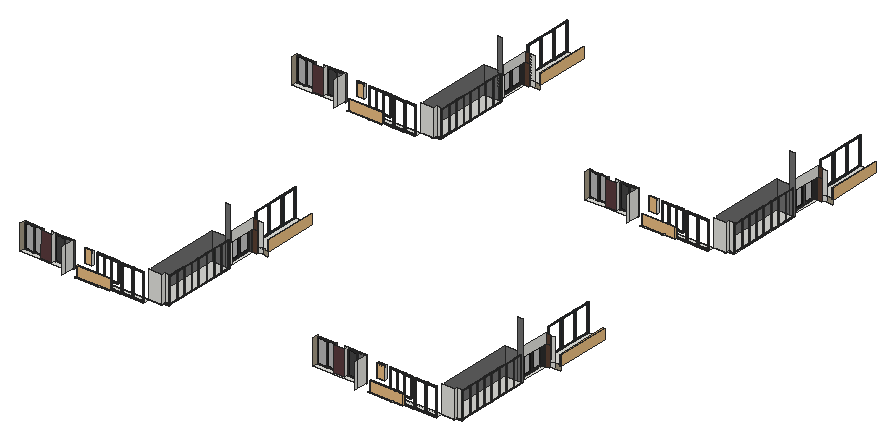
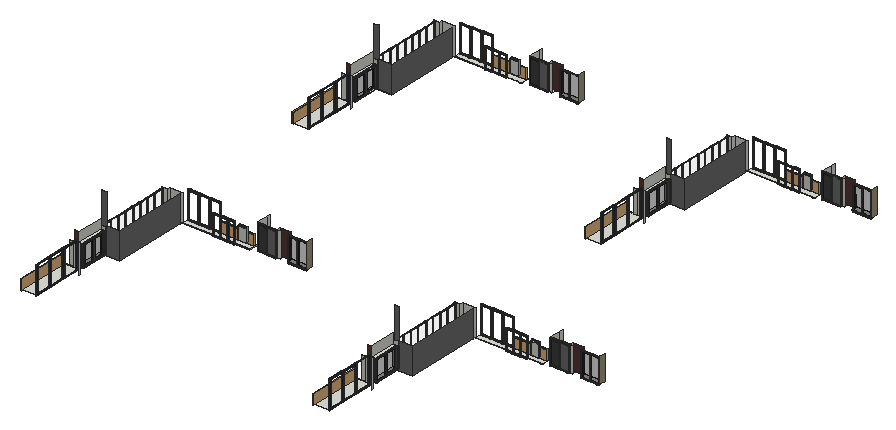
# SketchUp Ruby script. Lengths in inches.
U = 1.inch
M = Sketchup.active_model
def pt(a) = Geom::Point3d.new(a.map { |v| v * U })
def face(e, loops, mat)
  f = e.add_face(loops[0].map { |a| pt(a) })
  loops[1..].each { |l| e.add_face(l.map { |a| pt(a) }).erase! }
  f.material = f.back_material = mat if mat
  f
end
# faces: each face lists its corners as indices into pts; further lists are holes
def faces(e, pts, list, mat = nil) = list.each { |f| face(e, (f[0].is_a?(Array) ? f : [f]).map { |l| l.map { |i| pts[i] } }, mat) }
# xy, xz, yz: faces in a plane at the given z, y or x. An outline is a flat list of corners, or four numbers for a rectangle; further outlines are holes
def ring(l) = l.size == 4 ? [[l[0], l[1]], [l[2], l[1]], [l[2], l[3]], [l[0], l[3]]] : l.each_slice(2).to_a
def flat(e, list, mat, &to3) = list.each { |f| face(e, (f[0].is_a?(Array) ? f : [f]).map { |l| ring(l).map { |u, v| to3.(u, v) } }, mat) }
def xy(e, z, list, mat = nil) = flat(e, list, mat) { |x, y| [x, y, z] }
def xz(e, y, list, mat = nil) = flat(e, list, mat) { |x, z| [x, y, z] }
def yz(e, x, list, mat = nil) = flat(e, list, mat) { |y, z| [x, y, z] }
def lines(e, pts, list) = list.each { |a, b| e.add_line(pt(pts[a]), pt(pts[b])) }
# prism: a flat outline (further loops are holes) pulled along v
def prism(e, loops, v, mat = nil)
  f = face(e, loops, mat); d = Geom::Vector3d.new(v.map { |x| x * U })
  f.pushpull(f.normal.samedirection?(d) ? d.length : -d.length)
end
def box(e, o, s, mat = nil) = prism(e, [[o, [o[0] + s[0], o[1], o[2]], [o[0] + s[0], o[1] + s[1], o[2]], [o[0], o[1] + s[1], o[2]]]], [0, 0, s[2]], mat)
def at(x, y, z, deg = 0) = Geom::Transformation.translation(pt([x, y, z])) * Geom::Transformation.rotation(ORIGIN, Z_AXIS, deg.degrees)
def axes(o, x, y, z) = Geom::Transformation.new([*x, 0, *y, 0, *z, 0, *pt(o).to_a, 1])
def part(name) = M.definitions.add(name)
# library, detail: a bought-in or finely detailed component or shape, given as its bounding box
def library(name, o, s) = part(name).tap { |d| box(d.entities, o, s) }
def detail(e, o, s) = box(e.add_group.entities, o, s)
def put(e, d, t, mat = nil) = e.add_instance(d, t).tap { |i| i.material = mat if mat }
def group(e, t, mat = nil) = e.add_group.tap { |g| g.transformation = t; g.material = mat if mat }.entities
root = M.entities
M.materials.add("Glass_Tinted_Gray").color = [0, 0, 0]
M.materials["Glass_Tinted_Gray"].alpha = 0.125
M.materials.add("Glazing").color = [128, 128, 128]
M.materials["Glazing"].alpha = 0.05
M.materials.add("Powdercoating").color = [41, 44, 40]
M.materials.add("Wine2").color = [0, 0, 0]
M.materials["Wine2"].alpha = 0
M.materials.add("[0130_Gainsboro]").color = [39, 45, 50]
M.materials.add("[0135_DarkGray]").color = [81, 81, 81]
M.materials.add("[Color M05]").color = [114, 114, 114]
M.materials.add("[Color M06]").color = [86, 86, 86]
M.materials.add("[Concrete Tile]").color = [165, 155, 133]
M.materials.add("[Granite Brown]").color = [89, 59, 61]
M.materials.add("[Granite Brown]1").color = [89, 63, 50]
M.materials.add("[Mirror 02]").color = [229, 229, 229]
M.materials.add("[Terrazzo Light Blue]").color = [196, 214, 227]
c1 = library("Glass Railing",[0,0,0],[139.5,4.76,42])
c2 = part("Framed glazing panel")
xy(c2.entities,0,[[0,-0.98,43.07,0],[0,0,43.07,1.4]],"[0130_Gainsboro]")
xy(c2.entities,0.3,[[0.3,-1.43,42.77,-0.98]],"[0130_Gainsboro]")
xy(c2.entities,2.95,[[2.95,-1.43,40.12,-0.63],[2.95,-0.63,40.12,0],[2.95,0,40.12,0.64],[2.95,0.64,40.12,1.4]],"[0130_Gainsboro]")
xy(c2.entities,3.54,[[3.54,-0.63,39.53,0],[3.54,0,39.53,0.64]],"[0130_Gainsboro]")
xy(c2.entities,111.8125,[[3.54,-0.63,39.53,0],[3.54,0,39.53,0.64]],"[0130_Gainsboro]")
xy(c2.entities,112.4,[[2.95,-1.43,40.12,-0.63],[2.95,-0.63,40.12,0],[2.95,0,40.12,0.64],[2.95,0.64,40.12,1.4]],"[0130_Gainsboro]")
xy(c2.entities,115.05,[[0.3,-1.43,42.77,-0.98]],"[0130_Gainsboro]")
xy(c2.entities,115.35,[[0,-0.98,43.07,0],[0,0,43.07,1.4]],"[0130_Gainsboro]")
xz(c2.entities,-1.43,[[[0.3,0.3,42.77,115.05],[2.95,2.95,40.12,112.4]]],"[0130_Gainsboro]")
xz(c2.entities,-0.98,[[[0,0,43.07,115.35],[0.3,0.3,42.77,115.05]]],"[0130_Gainsboro]")
xz(c2.entities,-0.63,[[[2.95,2.95,40.12,112.4],[3.54,3.54,39.53,111.8125]]],"[0130_Gainsboro]")
xz(c2.entities,0,[[3.54,3.54,39.53,111.8125]],"Wine2")
xz(c2.entities,0,[[[0,0,43.07,115.35],[2.95,2.95,40.12,112.4]],[[2.95,2.95,40.12,112.4],[3.54,3.54,39.53,111.8125]]],"[0130_Gainsboro]")
xz(c2.entities,0.64,[[[2.95,2.95,40.12,112.4],[3.54,3.54,39.53,111.8125]]],"[0130_Gainsboro]")
xz(c2.entities,1.4,[[[0,0,43.07,115.35],[2.95,2.95,40.12,112.4]]],"[0130_Gainsboro]")
yz(c2.entities,0,[[-0.98,0,0,115.35],[0,0,1.4,115.35]],"[0130_Gainsboro]")
yz(c2.entities,0.3,[[-1.43,0.3,-0.98,115.05]],"[0130_Gainsboro]")
yz(c2.entities,2.95,[[-1.43,2.95,-0.63,112.4],[-0.63,2.95,0,112.4],[0,2.95,0.64,112.4],[0.64,2.95,1.4,112.4]],"[0130_Gainsboro]")
yz(c2.entities,3.54,[[-0.63,3.54,0,111.8125],[0,3.54,0.64,111.8125]],"[0130_Gainsboro]")
yz(c2.entities,39.53,[[-0.63,3.54,0,111.8125],[0,3.54,0.64,111.8125]],"[0130_Gainsboro]")
yz(c2.entities,40.12,[[-1.43,2.95,-0.63,112.4],[-0.63,2.95,0,112.4],[0,2.95,0.64,112.4],[0.64,2.95,1.4,112.4]],"[0130_Gainsboro]")
yz(c2.entities,42.77,[[-1.43,0.3,-0.98,115.05]],"[0130_Gainsboro]")
yz(c2.entities,43.07,[[-0.98,0,0,115.35],[0,0,1.4,115.35]],"[0130_Gainsboro]")
c3 = part("Glazed panel assembly")
put(c3.entities,c2,axes([90.57,1.43,0],[1.05148,0,0],[0,1,0],[0,0,1]))
put(c3.entities,c2,axes([0,1.43,0],[1.05148,0,0],[0,1,0],[0,0,1]))
put(c3.entities,c2,axes([45.29,1.43,0],[1.05148,0,0],[0,1,0],[0,0,1]))
c4 = part("Group\#15")
xy(c4.entities,0,[[0,-55.94,0.71,45.94]])
xy(c4.entities,0.2,[[0,-55.94,0.47,45.94],[0.47,45.94,0.71,46.42]])
xy(c4.entities,2.36,[[0.47,-55.94,0.71,46.42]])
xz(c4.entities,-55.94,[[0,0,0.71,0,0.71,2.36,0.47,2.36,0.47,0.2,0,0.2]])
xz(c4.entities,45.94,[[0,0,0.71,0.2]])
xz(c4.entities,46.42,[[0.47,0.2,0.71,2.36]])
yz(c4.entities,0,[[-55.94,0,45.94,0.2]])
yz(c4.entities,0.47,[[-55.94,0.2,46.42,2.36]])
yz(c4.entities,0.71,[[-55.94,0,45.94,0,45.94,0.2,46.42,0.2,46.42,2.36,-55.94,2.36]])
c5 = part("Group\#7")
xy(c5.entities,0,[[0,-59.09,0.71,45.94]])
xy(c5.entities,0.2,[[0,-59.09,0.47,45.94],[0.47,45.94,0.71,46.42]])
xy(c5.entities,2.36,[[0.47,-59.09,0.71,46.42]])
xz(c5.entities,-59.09,[[0,0,0.71,0,0.71,2.36,0.47,2.36,0.47,0.2,0,0.2]])
xz(c5.entities,45.94,[[0,0,0.71,0.2]])
xz(c5.entities,46.42,[[0.47,0.2,0.71,2.36]])
yz(c5.entities,0,[[-59.09,0,45.94,0.2]])
yz(c5.entities,0.47,[[-59.09,0.2,46.42,2.36]])
yz(c5.entities,0.71,[[-59.09,0,45.94,0,45.94,0.2,46.42,0.2,46.42,2.36,-59.09,2.36]])
c6 = part("Group\#16")
prism(c6.entities,[[[0.47,-56.18,0.2],[0,-56.18,0.2],[0,-56.18,0],[0.71,-56.18,0],[0.71,-56.18,2.36],[0.47,-56.18,2.36]]],[0,28.68,0])
c7 = part("Group\#10")
box(c7.entities,[-0.73,0,0],[27.99,0.55,102.05])
c8 = part("Group\#18")
xy(c8.entities,0,[[0.47,-56.18,0.47,-55.47,0,-55.47,0,-28.21,1.18,-28.21,1.18,-56.18]])
xy(c8.entities,0.2,[[0.71,-56.18,1.18,-28.21],[0,-55.47,0.47,-28.21],[0.47,-28.21,0.71,-27.74]])
xy(c8.entities,2.36,[[0.47,-56.18,0.71,-27.74]])
xz(c8.entities,-56.18,[[0.47,0,1.18,0,1.18,0.2,0.71,0.2,0.71,2.36,0.47,2.36]])
xz(c8.entities,-55.47,[[0,0,0.47,0.2]])
xz(c8.entities,-28.21,[[0,0,1.18,0.2]])
xz(c8.entities,-27.74,[[0.47,0.2,0.71,2.36]])
yz(c8.entities,0,[[-55.47,0,-28.21,0.2]])
yz(c8.entities,0.47,[[-56.18,0,-55.47,0.2],[-56.18,0.2,-27.74,2.36]])
yz(c8.entities,0.71,[[-56.18,0.2,-27.74,2.36]])
yz(c8.entities,1.18,[[-56.18,0,-28.21,0.2]])
c9 = part("Group\#34")
xy(c9.entities,0,[[-20.45,0,7.76,1.22]])
xy(c9.entities,0.06,[[-20.39,0.06,7.7,1.22]])
xy(c9.entities,0.47,[[-19.98,0,7.28,0.06]])
xy(c9.entities,101.89,[[-19.98,0,7.28,0.06]])
xy(c9.entities,102.3,[[-20.39,0.06,7.7,1.22]])
xy(c9.entities,102.36,[[-20.45,0,7.76,1.22]])
xz(c9.entities,0,[[[-20.45,0,7.76,102.36],[-19.98,0.47,7.28,101.89]]])
xz(c9.entities,0.06,[[[-20.39,0.06,7.7,102.3],[-19.98,0.47,7.28,101.89]]])
xz(c9.entities,1.22,[[[-20.45,0,7.76,102.36],[-20.39,0.06,7.7,102.3]]])
yz(c9.entities,-20.45,[[0,0,1.22,102.36]])
yz(c9.entities,-20.39,[[0.06,0.06,1.22,102.3]])
yz(c9.entities,-19.98,[[0,0.47,0.06,101.89]])
yz(c9.entities,7.28,[[0,0.47,0.06,101.89]])
yz(c9.entities,7.7,[[0.06,0.06,1.22,102.3]])
yz(c9.entities,7.76,[[0,0,1.22,102.36]])
c10 = part("Group\#6")
put(c10.entities,c4,axes([27.97,0,7.875],[1,0,0],[0,0,-1],[0,1,0]),"Powdercoating")
put(c10.entities,c5,axes([0.71,0,6.8],[-1,0,0],[0,0,-0.97687],[0,1,0]),"Powdercoating")
put(c10.entities,c6,axes([-27.5,0,-38.07],[0,0,-1],[-1,0,0],[0,1,0]),"Powdercoating")
put(c10.entities,c7,at(1.12,0.35,-38.39),"Glazing")
put(c10.entities,c8,axes([-27.5,0,63.35],[0,0,1],[-1,0,0],[0,1,0]),"Powdercoating")
put(c10.entities,c9,at(20.6875,1.0625,-38.54),"Powdercoating")
c11 = part("Sliding door assembly")
put(c11.entities,c10,at(-1.18,4.5,38.86))
g1 = group(c11.entities,at(84.74,4.5,38.86))
put(g1,c4,axes([-27.97,0,7.875],[-1,0,0],[0,0,-1],[0,1,0]),"Powdercoating")
put(g1,c5,axes([-0.71,0,6.8],[1,0,0],[0,0,-0.97687],[0,1,0]),"Powdercoating")
put(g1,c6,axes([27.5,0,-38.07],[0,0,-1],[1,0,0],[0,1,0]),"Powdercoating")
put(g1,c7,axes([-1.12,0.35,-38.39],[-1,0,0],[0,1,0],[0,0,1]),"Glazing")
put(g1,c8,axes([27.5,0,63.35],[0,0,1],[1,0,0],[0,1,0]),"Powdercoating")
put(g1,c9,axes([-20.6875,1.0625,-38.54],[-1,0,0],[0,1,0],[0,0,1]),"Powdercoating")
g2 = group(c11.entities,at(56.0625,4.5,38.86))
put(g2,c4,axes([-27.97,0,7.875],[-1,0,0],[0,0,-1],[0,1,0]),"Powdercoating")
put(g2,c6,axes([27.5,0,-38.07],[0,0,-1],[1,0,0],[0,1,0]),"Powdercoating")
put(g2,c7,axes([-1.12,0.35,-38.39],[-1,0,0],[0,1,0],[0,0,1]),"Glazing")
put(g2,c8,axes([27.5,0,63.35],[0,0,1],[1,0,0],[0,1,0]),"Powdercoating")
put(g2,c9,axes([-20.6875,1.0625,-38.54],[-1,0,0],[0,1,0],[0,0,1]),"Powdercoating")
g3 = group(g2,at(-0.71,0,6.8),"Powdercoating")
xy(g3,-45.34,[[0.47,0.2,0.71,2.36]])
xy(g3,-44.88,[[0,0,0.71,0.2]])
xy(g3,57.73,[[0,0,0.71,0,0.71,2.36,0.47,2.36,0.47,0.2,0,0.2]])
xz(g3,0,[[0,-44.88,0.71,57.73]])
xz(g3,0.2,[[0.47,-45.34,0.71,-44.88],[0,-44.88,0.47,57.73]])
xz(g3,2.36,[[0.47,-45.34,0.71,57.73]])
yz(g3,0,[[0,-44.88,0.2,57.73]])
yz(g3,0.47,[[0.2,-45.34,2.36,57.73]])
yz(g3,0.71,[[0.2,-45.34,2.36,-45.34,2.36,57.73,0,57.73,0,-44.88,0.2,-44.88]])
put(c11.entities,c10,axes([-33.94,4.5,38.86],[1.14218,0,0],[0,1,0],[0,0,1]))
c12 = part("sliding door")
put(c12.entities,c11,at(0,-4.5,-0.08))
c13 = part("PENTEK_RP Fineline 50S_Sliding_DoorCase_E1")
box(c13.entities,[0,0,0],[1.51,3.66,99.27],"[0135_DarkGray]")
c14 = part("PENTEK_RP Fineline 50S_SlidingDooe_Case_E2")
box(c14.entities,[0,0,0],[96.25,3.66,1.51],"[0135_DarkGray]")
c15 = part("pentek_RP Fineline 50S_SlidingDoor_Case")
put(c15.entities,c13,at(97.76,0,0))
put(c15.entities,c14,at(1.51,0,0))
put(c15.entities,c13,at(0,0,0))
put(c15.entities,c14,at(1.51,0,97.76))
c16 = part("PENTEK_RP Fineline 50S_SlidingDoor_GlazingBead_2")
box(c16.entities,[0,0,0],[0.56,0.59,94.39],"[0135_DarkGray]")
c17 = part("PENTEK_RP Fineline 50S_SlidingDoor_Glass")
box(c17.entities,[0,0,0],[46.58,0.16,94.39],"Glass_Tinted_Gray")
c18 = part("PENTEK_RP Fineline 50S_SlidingDoor_GlazingBead")
box(c18.entities,[0,0,0],[45.47,0.59,0.56],"[0135_DarkGray]")
c19 = part("PENTEK_RP Fineline 50S_SlidingDoor_Leaf_E1")
xy(c19.entities,0,[[0,0,0.93,1.97],[0.93,1.57,1.49,1.97]],"[0135_DarkGray]")
xy(c19.entities,96.25,[[0,0,0.93,0,0.93,1.57,1.49,1.57,1.49,1.97,0,1.97]],"[0135_DarkGray]")
xz(c19.entities,0,[[0,0,0.93,96.25]],"[0135_DarkGray]")
xz(c19.entities,1.57,[[0.93,0,1.49,95.32],[0.93,95.32,1.49,96.25]],"[0135_DarkGray]")
xz(c19.entities,1.97,[[0,0,1.49,96.25]],"[0135_DarkGray]")
yz(c19.entities,0,[[0,0,1.97,96.25]],"[0135_DarkGray]")
yz(c19.entities,0.93,[[0,0,1.57,0.93],[0,0.93,1.57,95.32],[0,95.32,1.57,96.25]],"[0135_DarkGray]")
yz(c19.entities,1.49,[[1.57,0,1.97,95.32],[1.57,95.32,1.97,96.25]],"[0135_DarkGray]")
c20 = part("PENTEK_RP Fineline 50S_SlidingDoor_Leaf_E2")
xy(c20.entities,0,[[0,0,0,1.57,0.56,1.57,0.56,1.97,46.02,1.97,46.02,1.57,46.58,1.57,46.58,0]],"[0135_DarkGray]")
xy(c20.entities,0.93,[[0,0,46.58,1.57]],"[0135_DarkGray]")
xy(c20.entities,1.49,[[0.56,1.57,46.02,1.97]],"[0135_DarkGray]")
xz(c20.entities,0,[[0,0,46.58,0.93]],"[0135_DarkGray]")
xz(c20.entities,1.57,[[0,0,0.56,0.93],[46.02,0,46.58,0.93],[0.56,0.93,46.02,1.49]],"[0135_DarkGray]")
xz(c20.entities,1.97,[[0.56,0,46.02,1.49]],"[0135_DarkGray]")
yz(c20.entities,0,[[0,0,1.57,0.93]],"[0135_DarkGray]")
yz(c20.entities,0.56,[[1.57,0,1.97,0.93],[1.57,0.93,1.97,1.49]],"[0135_DarkGray]")
yz(c20.entities,46.02,[[1.57,0,1.97,0.93],[1.57,0.93,1.97,1.49]],"[0135_DarkGray]")
yz(c20.entities,46.58,[[0,0,1.57,0.93]],"[0135_DarkGray]")
c21 = part("PENTEK_RP Fineline S_SlidingDoor_Leaf1")
put(c21.entities,c16,at(0.93,0,0.93))
put(c21.entities,c16,at(46.96,0,0.93))
put(c21.entities,c17,at(1.49,1.42,0.93))
put(c21.entities,c18,at(1.49,0,0.93))
put(c21.entities,c17,at(1.49,0.59,0.93),"[Terrazzo Light Blue]")
put(c21.entities,c19,at(0,0,0))
put(c21.entities,c19,axes([48.44,0,0],[-1,0,0],[0,1,0],[0,0,1]))
put(c21.entities,c20,axes([0.93,0,96.25],[1,0,0],[0,1,0],[0,0,-1]))
put(c21.entities,c20,at(0.93,0,0))
put(c21.entities,c18,at(1.49,0,94.77))
c22 = part("PENTEK_RP Fineline 50S_SlidingDoor_Leaf2")
put(c22.entities,c17,at(1.49,1.42,0.93))
put(c22.entities,c18,at(1.49,0,94.77))
put(c22.entities,c16,at(46.96,0,0.93))
put(c22.entities,c17,at(1.49,0.59,0.93),"[Mirror 02]")
put(c22.entities,c16,at(0.93,0,0.93))
put(c22.entities,c19,at(0,0,0))
put(c22.entities,c19,axes([48.44,0,0],[-1,0,0],[0,1,0],[0,0,1]))
put(c22.entities,c18,at(1.49,0,0.93))
put(c22.entities,c20,axes([0.93,0,96.25],[1,0,0],[0,1,0],[0,0,-1]))
put(c22.entities,c20,at(0.93,0,0))
c23 = part("PENTEK - Slimmest Steel Sliding Door / Window\#1")
put(c23.entities,c15,at(0,-1.88,-0.09))
put(c23.entities,c21,at(1.51,-2.27,1.42))
put(c23.entities,c22,at(49.32,-0.3,1.42))
c24 = library("Klein+raam",[128.36,12.7,0],[19.68,5.51,55.12])
xy(root,516.375,[[657.21,1788.5,701.53,1795.6875],[1875.4,1788.5,1919.71,1795.6875],[657.21,3203.1875,701.53,3210.375],[1875.4,3203.1875,1919.71,3210.375]])
xy(root,517.25,[[557.88,1788.5,657.21,1788.5,657.21,1795.6875,835.99,1795.6875,835.99,1822.9375,557.88,1822.9375],[1776.07,1788.5,1875.4,1788.5,1875.4,1795.6875,2054.17,1795.6875,2054.17,1822.9375,1776.07,1822.9375],[838.125,1835.1875,913.875,2148.83],[2056.3125,1835.1875,2132.0625,2148.83],[557.88,3203.1875,657.21,3203.1875,657.21,3210.375,835.99,3210.375,835.99,3237.625,557.88,3237.625],
  [1776.07,3203.1875,1875.4,3203.1875,1875.4,3210.375,2054.17,3210.375,2054.17,3237.625,1776.07,3237.625],[838.125,3249.875,913.875,3563.51],[2056.3125,3249.875,2132.0625,3563.51]])
xy(root,517.25,[[557.4,1788.5,557.88,1822.9375],[1775.59,1788.5,1776.07,1822.9375],[557.4,3203.1875,557.88,3237.625],[1775.59,3203.1875,1776.07,3237.625]],"[Granite Brown]")
xy(root,525.4375,[[319.53,1799.9375,401.17,1822.9375],[401.17,1799.9375,431.33,1806.5625],[431.33,1799.9375,523.04,1799.9375,523.04,1822.9375,446.15,1822.9375,446.15,1806.5625,431.33,1806.5625],[1537.72,1799.9375,1619.36,1822.9375],[1619.36,1799.9375,1649.52,1806.5625],
  [1649.52,1799.9375,1741.23,1799.9375,1741.23,1822.9375,1664.33,1822.9375,1664.33,1806.5625,1649.52,1806.5625],[431.33,1806.5625,446.15,1822.9375],[1649.52,1806.5625,1664.33,1822.9375],[319.53,3214.625,401.17,3237.625],[401.17,3214.625,431.33,3221.25],
  [431.33,3214.625,523.04,3214.625,523.04,3237.625,446.15,3237.625,446.15,3221.25,431.33,3221.25],[1537.72,3214.625,1619.36,3237.625],[1619.36,3214.625,1649.52,3221.25],[1649.52,3214.625,1741.23,3214.625,1741.23,3237.625,1664.33,3237.625,1664.33,3221.25,1649.52,3221.25],[431.33,3221.25,446.15,3237.625],
  [1649.52,3221.25,1664.33,3237.625]])
xy(root,527.36,[[890.875,2156.01,913.875,2266.33],[2109.0625,2156.01,2132.0625,2266.33],[890.875,3570.7,913.875,3681.01],[2109.0625,3570.7,2132.0625,3681.01]])
xy(root,534.0625,[[890.875,2295.875,954.6875,2518.89],[2109.0625,2295.875,2172.875,2518.89],[890.875,3710.5625,954.6875,3933.57],[2109.0625,3710.5625,2172.875,3933.57]])
xy(root,551.24,[[557.88,1835.1875,589.71,1845.8125],[1776.07,1835.1875,1807.9,1845.8125],[557.88,3249.875,589.71,3260.5],[1776.07,3249.875,1807.9,3260.5]])
xy(root,603.53,[[557.88,1835.1875,589.71,1845.8125],[1776.07,1835.1875,1807.9,1845.8125],[557.88,3249.875,589.71,3260.5],[1776.07,3249.875,1807.9,3260.5]])
xy(root,608.125,[[611.65,1835.1875,701.59,1837.0625],[1829.84,1835.1875,1919.77,1837.0625],[611.65,3249.875,701.59,3251.75],[1829.84,3249.875,1919.77,3251.75]])
xy(root,613.04,[[890.875,2156.01,913.875,2266.33],[2109.0625,2156.01,2132.0625,2266.33],[890.875,3570.7,913.875,3681.01],[2109.0625,3570.7,2132.0625,3681.01]])
xz(root,1788.5,[[557.88,516.375,657.21,517.25],[1776.07,516.375,1875.4,517.25]])
xz(root,1788.5,[[557.4,516.375,557.88,517.25],[1775.59,516.375,1776.07,517.25]],"[Granite Brown]")
xz(root,1806.5625,[[401.25,525.4375,446.15,525.4375,446.15,630,401.77,630],[1619.4375,525.4375,1664.33,525.4375,1664.33,630,1619.96,630]],"[Granite Brown]")
xz(root,1822.9375,[[557.88,516.375,632.49,517.25],[632.49,516.375,890.875,517.25],[1776.07,516.375,1850.67,517.25],[1850.67,516.375,2109.0625,517.25],[835.99,517.25,890.875,630],
  [2054.17,517.25,2109.0625,630],[431.33,525.4375,446.15,630],[1649.52,525.4375,1664.33,630]])
xz(root,1822.9375,[[446.15,525.4375,523.04,630],[1664.33,525.4375,1741.23,630]],"[Color M05]")
xz(root,1822.9375,[[557.4,516.375,557.88,517.25],[1775.59,516.375,1776.07,517.25]],"[Granite Brown]")
xz(root,1835.1875,[[890.875,516.375,913.875,517.25],[2109.0625,516.375,2132.0625,517.25],[890.875,517.25,913.875,517.3125],[2109.0625,517.25,2132.0625,517.3125],[890.875,517.3125,913.875,630],
  [2109.0625,517.3125,2132.0625,630]])
xz(root,1845.8125,[[557.88,551.24,589.71,603.53],[1776.07,551.24,1807.9,603.53]])
xz(root,2148.83,[[838.125,517.25,894.3125,630],[894.3125,517.25,913.875,756],[2056.3125,517.25,2112.5,630],[2112.5,517.25,2132.0625,756]],"[Color M05]")
xz(root,2156.01,[[890.875,527.36,894.3125,613.04],[894.3125,527.36,913.875,613.04],[2109.0625,527.36,2112.5,613.04],[2112.5,527.36,2132.0625,613.04],[894.3125,613.04,913.875,630],
  [2112.5,613.04,2132.0625,630]])
xz(root,2266.33,[[913.875,527.36,930.75,613.04],[2132.0625,527.36,2148.9375,613.04],[913.875,613.04,930.75,653.36],[2132.0625,613.04,2148.9375,653.36]],"[Granite Brown]1")
xz(root,2295.875,[[913.875,511.75,930.75,534.0625],[2132.0625,511.75,2148.9375,534.0625],[890.875,534.0625,913.875,630],[913.875,534.0625,930.75,630],[2109.0625,534.0625,2132.0625,630],
  [2132.0625,534.0625,2148.9375,630]])
xz(root,2295.875,[[930.75,511.75,954.6875,534.0625],[2148.9375,511.75,2172.875,534.0625]],"[Concrete Tile]")
xz(root,3203.1875,[[557.88,516.375,657.21,517.25],[1776.07,516.375,1875.4,517.25]])
xz(root,3203.1875,[[557.4,516.375,557.88,517.25],[1775.59,516.375,1776.07,517.25]],"[Granite Brown]")
xz(root,3221.25,[[401.25,525.4375,446.15,525.4375,446.15,630,401.77,630],[1619.4375,525.4375,1664.33,525.4375,1664.33,630,1619.96,630]],"[Granite Brown]")
xz(root,3237.625,[[557.88,516.375,632.49,517.25],[632.49,516.375,890.875,517.25],[1776.07,516.375,1850.67,517.25],[1850.67,516.375,2109.0625,517.25],[835.99,517.25,890.875,630],
  [2054.17,517.25,2109.0625,630],[431.33,525.4375,446.15,630],[1649.52,525.4375,1664.33,630]])
xz(root,3237.625,[[446.15,525.4375,523.04,630],[1664.33,525.4375,1741.23,630]],"[Color M05]")
xz(root,3237.625,[[557.4,516.375,557.88,517.25],[1775.59,516.375,1776.07,517.25]],"[Granite Brown]")
xz(root,3249.875,[[890.875,516.375,913.875,517.25],[2109.0625,516.375,2132.0625,517.25],[890.875,517.25,913.875,517.3125],[2109.0625,517.25,2132.0625,517.3125],[890.875,517.3125,913.875,630],
  [2109.0625,517.3125,2132.0625,630]])
xz(root,3260.5,[[557.88,551.24,589.71,603.53],[1776.07,551.24,1807.9,603.53]])
xz(root,3563.51,[[838.125,517.25,894.3125,630],[894.3125,517.25,913.875,756],[2056.3125,517.25,2112.5,630],[2112.5,517.25,2132.0625,756]],"[Color M05]")
xz(root,3570.7,[[890.875,527.36,894.3125,613.04],[894.3125,527.36,913.875,613.04],[2109.0625,527.36,2112.5,613.04],[2112.5,527.36,2132.0625,613.04],[894.3125,613.04,913.875,630],
  [2112.5,613.04,2132.0625,630]])
xz(root,3681.01,[[913.875,527.36,930.75,613.04],[2132.0625,527.36,2148.9375,613.04],[913.875,613.04,930.75,653.36],[2132.0625,613.04,2148.9375,653.36]],"[Granite Brown]1")
xz(root,3710.5625,[[913.875,511.75,930.75,534.0625],[2132.0625,511.75,2148.9375,534.0625],[890.875,534.0625,913.875,630],[913.875,534.0625,930.75,630],[2109.0625,534.0625,2132.0625,630],
  [2132.0625,534.0625,2148.9375,630]])
xz(root,3710.5625,[[930.75,511.75,954.6875,534.0625],[2148.9375,511.75,2172.875,534.0625]],"[Concrete Tile]")
yz(root,319.53,[[1799.9375,525.4375,1822.9375,630],[3214.625,525.4375,3237.625,630]],"[Concrete Tile]")
yz(root,446.15,[[1806.5625,525.4375,1822.9375,630],[3221.25,525.4375,3237.625,630]])
yz(root,523.04,[[1763.25,525.4375,1822.9375,630],[3177.9375,525.4375,3237.625,630]])
yz(root,557.4,[[1788.5,516.375,1822.9375,517.25],[3203.1875,516.375,3237.625,517.25]])
yz(root,589.71,[[1835.1875,551.24,1845.8125,603.53],[3249.875,551.24,3260.5,603.53]])
yz(root,657.21,[[1788.5,516.375,1795.6875,517.25],[3203.1875,516.375,3210.375,517.25]])
yz(root,838.125,[[1835.1875,517.25,2148.83,630],[3249.875,517.25,3563.51,630]],"[Color M05]")
yz(root,890.875,[[2290,511.75,2295.875,630],[3704.6875,511.75,3710.5625,630],[1822.9375,516.375,1835.1875,517.25],[3237.625,516.375,3249.875,517.25],[1822.9375,517.25,1835.1875,517.3125],
  [3237.625,517.25,3249.875,517.3125],[1822.9375,517.3125,1835.1875,630],[3237.625,517.3125,3249.875,630]])
yz(root,913.875,[[2156.01,613.04,2266.33,653.36],[3570.7,613.04,3681.01,653.36]])
yz(root,1537.72,[[1799.9375,525.4375,1822.9375,630],[3214.625,525.4375,3237.625,630]],"[Concrete Tile]")
yz(root,1664.33,[[1806.5625,525.4375,1822.9375,630],[3221.25,525.4375,3237.625,630]])
yz(root,1741.23,[[1763.25,525.4375,1822.9375,630],[3177.9375,525.4375,3237.625,630]])
yz(root,1775.59,[[1788.5,516.375,1822.9375,517.25],[3203.1875,516.375,3237.625,517.25]])
yz(root,1807.9,[[1835.1875,551.24,1845.8125,603.53],[3249.875,551.24,3260.5,603.53]])
yz(root,1875.4,[[1788.5,516.375,1795.6875,517.25],[3203.1875,516.375,3210.375,517.25]])
yz(root,2056.3125,[[1835.1875,517.25,2148.83,630],[3249.875,517.25,3563.51,630]],"[Color M05]")
yz(root,2109.0625,[[2290,511.75,2295.875,630],[3704.6875,511.75,3710.5625,630],[1822.9375,516.375,1835.1875,517.25],[3237.625,516.375,3249.875,517.25],[1822.9375,517.25,1835.1875,517.3125],
  [3237.625,517.25,3249.875,517.3125],[1822.9375,517.3125,1835.1875,630],[3237.625,517.3125,3249.875,630]])
yz(root,2132.0625,[[2156.01,613.04,2266.33,653.36],[3570.7,613.04,3681.01,653.36]])
p = [[1850.67,1822.9375,517.25],[1850.67,1822.9375,517.3125],[2132.0625,1827.4375,517.3125],[2112.5,1827.4375,517.3125],[2112.5,1835.1875,517.3125],[2109.0625,1835.1875,517.3125],
  [2056.3125,1835.1875,517.3125],[1741.23,1778.3125,525.4375],[1741.23,1778.3125,630],[632.49,1822.9375,517.25],[632.49,1822.9375,517.3125],[913.875,1827.4375,517.3125],
  [894.3125,1827.4375,517.3125],[894.3125,1835.1875,517.3125],[890.875,1835.1875,517.3125],[838.125,1835.1875,517.3125],[523.04,1778.3125,525.4375],[523.04,1778.3125,630],
  [1741.23,3193,525.4375],[1741.23,3193,630],[2132.0625,3242.125,517.3125],[2112.5,3242.125,517.3125],[2112.5,3249.875,517.3125],[2109.0625,3249.875,517.3125],
  [2056.3125,3249.875,517.3125],[1850.67,3237.625,517.25],[1850.67,3237.625,517.3125],[913.875,3242.125,517.3125],[894.3125,3242.125,517.3125],[894.3125,3249.875,517.3125],
  [890.875,3249.875,517.3125],[838.125,3249.875,517.3125],[632.49,3237.625,517.25],[632.49,3237.625,517.3125],[523.04,3193,525.4375],[523.04,3193,630]]
lines(root,p,[[0,1],[2,3],[3,4],[5,6],[7,8],[9,10],[11,12],[12,13],[14,15],[16,17],[18,19],[20,21],
  [21,22],[23,24],[25,26],[27,28],[28,29],[30,31],[32,33],[34,35]])
put(root,c1,at(1779.13,1792.94,516.87))
put(root,c1,at(560.94,1792.94,516.87))
put(root,c1,at(1779.13,3207.63,516.87))
put(root,c1,at(560.94,3207.63,516.87))
put(root,c3,at(1918.3125,1795.6875,517.25))
put(root,c3,at(700.125,1795.6875,517.25))
put(root,c3,at(1918.3125,3210.375,517.25))
put(root,c3,at(700.125,3210.375,517.25))
put(root,c12,axes([2131,1878.45,517.99],[0,1.302,0],[-1,0,0],[0,0,1.03877]))
put(root,c12,axes([2131,2031.14,517.99],[0,1.302,0],[-1,0,0],[0,0,1.03877]))
put(root,c12,axes([912.8125,2031.14,517.99],[0,1.302,0],[-1,0,0],[0,0,1.03877]))
put(root,c12,axes([912.8125,1878.45,517.99],[0,1.302,0],[-1,0,0],[0,0,1.03877]))
put(root,c12,axes([2131,3293.14,517.99],[0,1.302,0],[-1,0,0],[0,0,1.03877]))
put(root,c12,axes([2131,3445.82,517.99],[0,1.302,0],[-1,0,0],[0,0,1.03877]))
put(root,c12,axes([912.8125,3293.14,517.99],[0,1.302,0],[-1,0,0],[0,0,1.03877]))
put(root,c12,axes([912.8125,3445.82,517.99],[0,1.302,0],[-1,0,0],[0,0,1.03877]))
put(root,c3,axes([1829.4375,1833.46,521.625],[0.6649,0,0],[0,0.61,0],[0,0,0.74986]),"[Color M06]")
put(root,c3,axes([611.25,1833.46,521.625],[0.6649,0,0],[0,0.61,0],[0,0,0.74986]),"[Color M06]")
put(root,c3,axes([1829.4375,3248.15,521.625],[0.6649,0,0],[0,0.61,0],[0,0,0.74986]),"[Color M06]")
put(root,c3,axes([611.25,3248.15,521.625],[0.6649,0,0],[0,0.61,0],[0,0,0.74986]),"[Color M06]")
put(root,c23,axes([1666.41,1823.2,522.375],[0.77709,0,0],[0,0.88,0],[0,0,1.054]))
put(root,c23,axes([1538.43,1823.2,522.375],[0.77709,0,0],[0,0.88,0],[0,0,1.054]))
put(root,c23,axes([320.24,1823.2,522.375],[0.77709,0,0],[0,0.88,0],[0,0,1.054]))
put(root,c23,axes([448.22,1823.2,522.375],[0.77709,0,0],[0,0.88,0],[0,0,1.054]))
put(root,c23,axes([1538.43,3237.89,522.375],[0.77709,0,0],[0,0.88,0],[0,0,1.054]))
put(root,c23,axes([1666.41,3237.89,522.375],[0.77709,0,0],[0,0.88,0],[0,0,1.054]))
put(root,c23,axes([448.22,3237.89,522.375],[0.77709,0,0],[0,0.88,0],[0,0,1.054]))
put(root,c23,axes([320.24,3237.89,522.375],[0.77709,0,0],[0,0.88,0],[0,0,1.054]))
put(root,c23,axes([2114.43,2158.32,525.29],[0,1.12181,0],[-2.51374,0,0],[0,0,0.87918]))
put(root,c23,axes([896.24,2158.32,525.29],[0,1.12181,0],[-2.51374,0,0],[0,0,0.87918]))
put(root,c23,axes([2114.43,3573.01,525.29],[0,1.12181,0],[-2.51374,0,0],[0,0,0.87918]))
put(root,c23,axes([896.24,3573.01,525.29],[0,1.12181,0],[-2.51374,0,0],[0,0,0.87918]))
put(root,c1,axes([2174.88,2295.6875,531.0625],[0,1.6,0],[-1,0,0],[0,0,1]))
put(root,c1,axes([956.7,2295.6875,531.0625],[0,1.6,0],[-1,0,0],[0,0,1]))
put(root,c1,axes([2174.88,3710.375,531.0625],[0,1.6,0],[-1,0,0],[0,0,1]))
put(root,c1,axes([956.7,3710.375,531.0625],[0,1.6,0],[-1,0,0],[0,0,1]))
put(root,c3,axes([2109.0625,2309.55,534.0625],[0,1.54079,0],[-1,0,0],[0,0,1]),"[Concrete Tile]")
put(root,c3,axes([890.875,2309.55,534.0625],[0,1.54079,0],[-1,0,0],[0,0,1]),"[Concrete Tile]")
put(root,c3,axes([2109.0625,3724.24,534.0625],[0,1.54079,0],[-1,0,0],[0,0,1]),"[Concrete Tile]")
put(root,c3,axes([890.875,3724.24,534.0625],[0,1.54079,0],[-1,0,0],[0,0,1]),"[Concrete Tile]")
put(root,c24,axes([1572.84,1826.55,551.24],[1.58777,0,0],[0,0.68,0],[0,0,0.99202]))
put(root,c24,axes([354.65,1826.55,551.24],[1.58777,0,0],[0,0.68,0],[0,0,0.99202]))
put(root,c24,axes([1572.84,3241.24,551.24],[1.58777,0,0],[0,0.68,0],[0,0,0.99202]))
put(root,c24,axes([354.65,3241.24,551.24],[1.58777,0,0],[0,0.68,0],[0,0,0.99202]))
